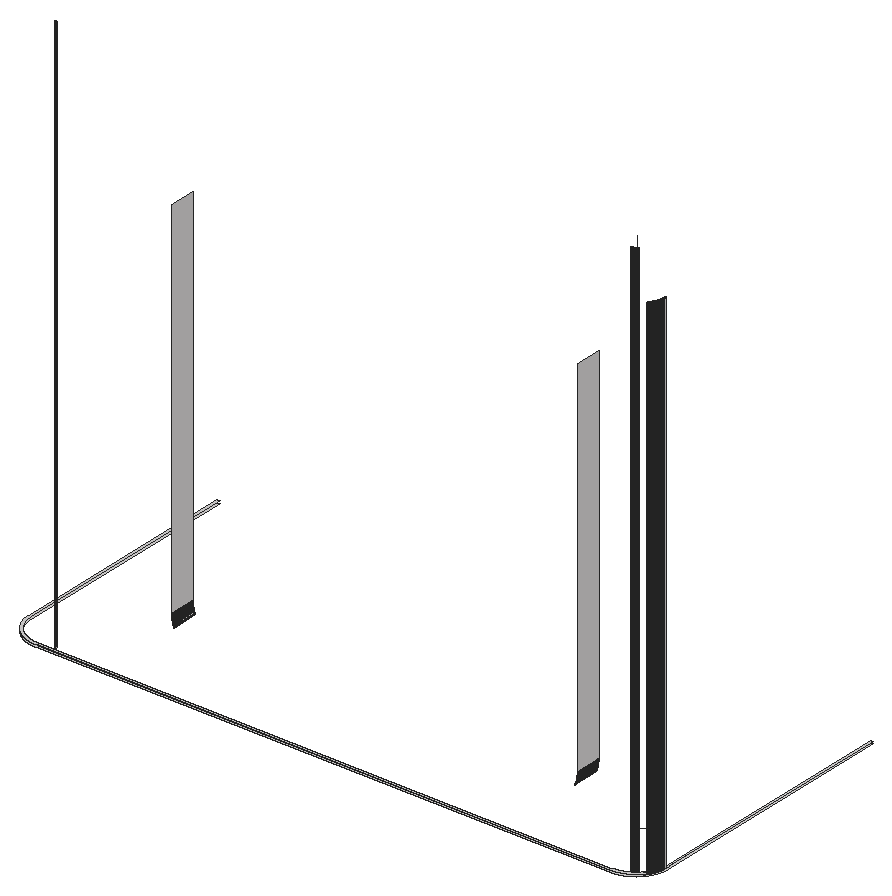
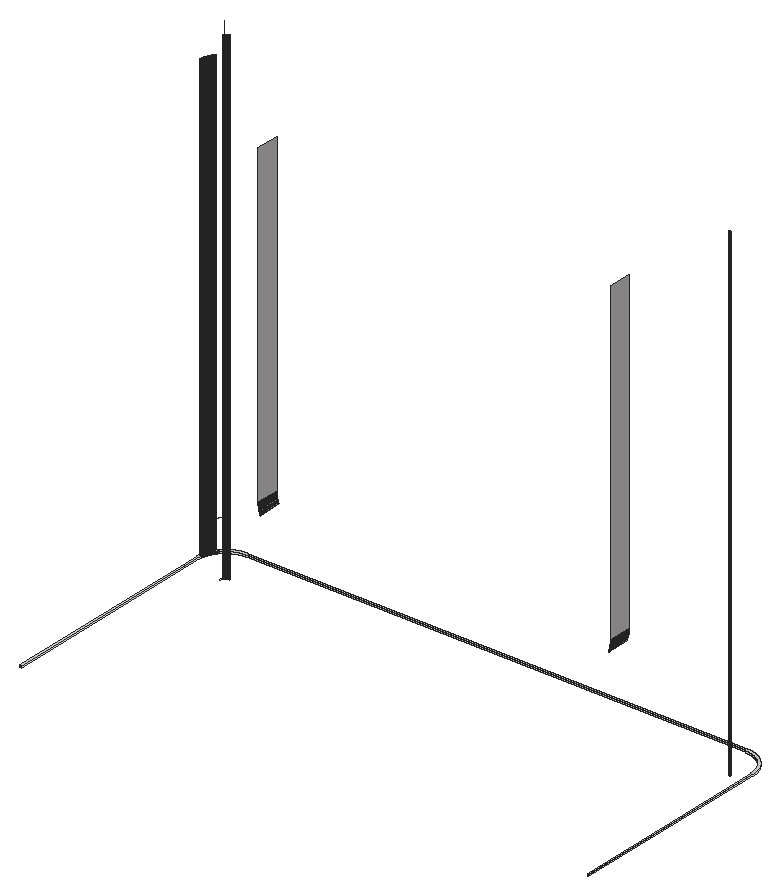
# SketchUp Ruby script. Lengths in inches.
U = 1.inch
M = Sketchup.active_model
def pt(a) = Geom::Point3d.new(a.map { |v| v * U })
def face(e, loops, mat)
  f = e.add_face(loops[0].map { |a| pt(a) })
  loops[1..].each { |l| e.add_face(l.map { |a| pt(a) }).erase! }
  f.material = f.back_material = mat if mat
  f
end
# faces: each face lists its corners as indices into pts; further lists are holes
def faces(e, pts, list, mat = nil) = list.each { |f| face(e, (f[0].is_a?(Array) ? f : [f]).map { |l| l.map { |i| pts[i] } }, mat) }
# xy, xz, yz: faces in a plane at the given z, y or x. An outline is a flat list of corners, or four numbers for a rectangle; further outlines are holes
def ring(l) = l.size == 4 ? [[l[0], l[1]], [l[2], l[1]], [l[2], l[3]], [l[0], l[3]]] : l.each_slice(2).to_a
def flat(e, list, mat, &to3) = list.each { |f| face(e, (f[0].is_a?(Array) ? f : [f]).map { |l| ring(l).map { |u, v| to3.(u, v) } }, mat) }
def xy(e, z, list, mat = nil) = flat(e, list, mat) { |x, y| [x, y, z] }
def xz(e, y, list, mat = nil) = flat(e, list, mat) { |x, z| [x, y, z] }
def yz(e, x, list, mat = nil) = flat(e, list, mat) { |y, z| [x, y, z] }
def lines(e, pts, list) = list.each { |a, b| e.add_line(pt(pts[a]), pt(pts[b])) }
# prism: a flat outline (further loops are holes) pulled along v
def prism(e, loops, v, mat = nil)
  f = face(e, loops, mat); d = Geom::Vector3d.new(v.map { |x| x * U })
  f.pushpull(f.normal.samedirection?(d) ? d.length : -d.length)
end
def box(e, o, s, mat = nil) = prism(e, [[o, [o[0] + s[0], o[1], o[2]], [o[0] + s[0], o[1] + s[1], o[2]], [o[0], o[1] + s[1], o[2]]]], [0, 0, s[2]], mat)
def at(x, y, z, deg = 0) = Geom::Transformation.translation(pt([x, y, z])) * Geom::Transformation.rotation(ORIGIN, Z_AXIS, deg.degrees)
def axes(o, x, y, z) = Geom::Transformation.new([*x, 0, *y, 0, *z, 0, *pt(o).to_a, 1])
def part(name) = M.definitions.add(name)
# library, detail: a bought-in or finely detailed component or shape, given as its bounding box
def library(name, o, s) = part(name).tap { |d| box(d.entities, o, s) }
def detail(e, o, s) = box(e.add_group.entities, o, s)
def put(e, d, t, mat = nil) = e.add_instance(d, t).tap { |i| i.material = mat if mat }
def group(e, t, mat = nil) = e.add_group.tap { |g| g.transformation = t; g.material = mat if mat }.entities
root = M.entities
M.materials.add("[Quartz Light Brown]").color = [215, 212, 212]
xy(root,126,[[480.082,155,480.118,155.002,480.196,155.006,480.235,155.009,480.275,155.013,480.311,155.016,480.314,155.016,480.392,155.026,480.425,155.03,480.43,155.031,480.508,155.043,480.538,155.048,480.547,155.05,480.585,155.058,480.624,155.066,480.651,155.071,480.662,155.074,480.738,155.092,480.762,155.098,480.776,155.102,480.852,155.124,480.873,155.129,480.89,155.135,480.964,155.159,480.982,155.165,481.001,155.172,481.038,155.185,481.075,155.199,481.089,155.204,481.112,155.214,481.148,155.228,481.184,155.244,481.196,155.248,481.22,155.259,481.256,155.276,481.292,155.292,481.3,155.296,481.327,155.309,481.397,155.345,481.402,155.348,481.431,155.364,481.466,155.383,481.5,155.402,481.503,155.403,481.534,155.422,481.567,155.442,481.601,155.463,481.634,155.484,481.697,155.526,481.699,155.528,481.731,155.55,481.763,155.573,481.79,155.592,481.795,155.596,481.857,155.644,481.881,155.663,481.888,155.669,481.918,155.693,481.948,155.719,481.969,155.736,481.978,155.744,482.007,155.771,482.036,155.797,482.054,155.813,482.065,155.824,482.093,155.851,482.121,155.879,482.136,155.893,482.149,155.907,482.176,155.935,482.203,155.964,482.215,155.977,482.229,155.993,482.256,156.022,482.281,156.052,482.291,156.063,482.307,156.082,482.331,156.112,482.356,156.143,482.364,156.152,482.38,156.174,482.404,156.205,482.427,156.237,482.432,156.244,482.45,156.269,482.494,156.333,482.498,156.338,482.516,156.366,482.537,156.399,482.558,156.433,482.56,156.435,482.578,156.466,482.598,156.5,482.617,156.534,482.636,156.569,482.655,156.603,482.672,156.635,482.673,156.638,482.691,156.673,482.708,156.708,482.722,156.738,482.724,156.744,482.741,156.78,482.756,156.816,482.772,156.852,482.786,156.888,482.801,156.925,482.81,156.95,482.815,156.962,482.841,157.036,482.849,157.058,482.853,157.073,482.865,157.11,482.876,157.148,482.882,157.168,482.887,157.186,482.898,157.224,482.908,157.262,482.912,157.279,482.917,157.3,482.926,157.338,482.934,157.376,482.9375,157.391,482.942,157.415,482.95,157.453,482.957,157.492,482.959,157.504,482.963,157.531,482.969,157.57,482.974,157.608,482.976,157.617,482.979,157.647,482.984,157.686,482.987,157.725,482.988,157.731,482.991,157.765,482.994,157.804,482.996,157.843,482.996,157.846,482.998,157.882,482.999,157.921,483,155]],"[Quartz Light Brown]")
xy(root,132,[[216,143,480,143,480.196,143.001,480.393,143.005,480.589,143.012,480.785,143.021,480.981,143.032,481.177,143.046,481.373,143.063,481.568,143.082,481.763,143.104,481.958,143.128,482.152,143.155,482.347,143.185,482.54,143.217,482.734,143.251,482.926,143.288,483.119,143.328,483.31,143.37,483.502,143.414,483.692,143.462,483.882,143.511,484.072,143.563,484.26,143.618,484.448,143.675,484.635,143.734,484.822,143.796,485.007,143.86,485.192,143.927,485.376,143.996,485.558,144.068,485.74,144.142,485.921,144.218,486.101,144.297,486.28,144.378,486.458,144.461,486.634,144.547,486.81,144.635,486.984,144.725,487.157,144.818,487.329,144.913,487.5,145.01,487.669,145.109,487.837,145.21,488.004,145.314,488.17,145.42,488.334,145.528,488.496,145.638,488.657,145.75,488.817,145.865,488.975,145.981,489.131,146.1,489.286,146.22,489.44,146.343,489.592,146.467,489.742,146.594,489.89,146.722,490.037,146.853,490.182,146.985,490.325,147.119,490.467,147.255,490.607,147.393,490.745,147.533,490.881,147.675,491.015,147.818,491.147,147.963,491.278,148.11,491.406,148.258,491.533,148.408,491.657,148.56,491.78,148.714,491.9,148.869,492.019,149.025,492.135,149.183,492.25,149.343,492.362,149.504,492.472,149.666,492.58,149.83,492.686,149.996,492.79,150.163,492.891,150.331,492.99,150.5,493.087,150.671,493.182,150.843,493.275,151.016,493.365,151.19,493.453,151.366,493.539,151.542,493.622,151.72,493.703,151.899,493.782,152.079,493.858,152.26,493.932,152.442,494.004,152.624,494.073,152.808,494.14,152.993,494.204,153.178,494.266,153.365,494.325,153.552,494.382,153.74,494.437,153.928,494.489,154.118,494.538,154.308,494.586,154.498,494.63,154.69,494.672,154.881,494.712,155.074,494.749,155.266,494.783,155.46,494.815,155.653,494.845,155.848,494.872,156.042,494.896,156.237,494.918,156.432,494.937,156.627,494.954,156.823,494.968,157.019,494.979,157.215,494.988,157.411,494.995,157.607,494.999,157.804,495,158,495,275,494,275,494,158.003,493.999,157.817,493.995,157.634,493.989,157.45,493.981,157.267,493.97,157.084,493.957,156.902,493.941,156.719,493.923,156.537,493.903,156.354,493.88,156.173,493.855,155.991,493.828,155.81,493.798,155.629,493.766,155.449,493.731,155.269,493.694,155.089,493.655,154.91,493.613,154.732,493.569,154.554,493.523,154.377,493.474,154.2,493.423,154.024,493.37,153.848,493.315,153.674,493.257,153.5,493.197,153.327,493.135,153.154,493.07,152.983,493.003,152.812,492.934,152.642,492.863,152.474,492.79,152.306,492.714,152.139,492.636,151.973,492.556,151.808,492.474,151.644,492.39,151.481,492.303,151.32,492.215,151.159,492.124,151,492.032,150.842,491.937,150.685,491.84,150.529,491.741,150.375,491.641,150.222,491.538,150.07,491.433,149.92,491.326,149.771,491.218,149.623,491.107,149.477,490.994,149.333,490.88,149.19,490.764,149.048,490.646,148.908,490.526,148.769,490.404,148.632,490.28,148.497,490.155,148.363,490.028,148.231,489.899,148.101,489.769,147.972,489.637,147.845,489.503,147.72,489.368,147.596,489.231,147.474,489.092,147.354,488.952,147.236,488.81,147.12,488.667,147.006,488.523,146.893,488.377,146.782,488.229,146.674,488.08,146.567,487.93,146.462,487.778,146.359,487.625,146.259,487.471,146.16,487.315,146.063,487.158,145.968,487,145.876,486.841,145.785,486.68,145.697,486.519,145.61,486.356,145.526,486.192,145.444,486.027,145.364,485.861,145.286,485.694,145.21,485.526,145.137,485.358,145.066,485.188,144.997,485.017,144.93,484.846,144.865,484.673,144.803,484.5,144.743,484.326,144.685,484.152,144.63,483.976,144.577,483.8,144.526,483.623,144.477,483.446,144.431,483.268,144.387,483.09,144.345,482.911,144.306,482.731,144.269,482.551,144.234,482.371,144.202,482.19,144.172,482.009,144.145,481.827,144.12,481.646,144.097,481.463,144.077,481.281,144.059,481.098,144.043,480.916,144.03,480.733,144.019,480.55,144.011,480.366,144.005,480.183,144.001,479.997,144,216.003,144,215.817,144.001,215.634,144.005,215.45,144.011,215.267,144.019,215.084,144.03,214.902,144.043,214.719,144.059,214.537,144.077,214.354,144.097,214.173,144.12,213.991,144.145,213.81,144.172,213.629,144.202,213.449,144.234,213.269,144.269,213.089,144.306,212.91,144.345,212.732,144.387,212.554,144.431,212.377,144.477,212.2,144.526,212.024,144.577,211.848,144.63,211.674,144.685,211.5,144.743,211.327,144.803,211.154,144.865,210.983,144.93,210.812,144.997,210.642,145.066,210.474,145.137,210.306,145.21,210.139,145.286,209.973,145.364,209.808,145.444,209.644,145.526,209.481,145.61,209.32,145.697,209.159,145.785,209,145.876,208.842,145.968,208.685,146.063,208.529,146.16,208.375,146.259,208.222,146.359,208.07,146.462,207.92,146.567,207.771,146.674,207.623,146.782,207.477,146.893,207.333,147.006,207.19,147.12,207.048,147.236,206.908,147.354,206.769,147.474,206.632,147.596,206.497,147.72,206.363,147.845,206.231,147.972,206.101,148.101,205.972,148.231,205.845,148.363,205.72,148.497,205.596,148.632,205.474,148.769,205.354,148.908,205.236,149.048,205.12,149.19,205.006,149.333,204.893,149.477,204.782,149.623,204.674,149.771,204.567,149.92,204.462,150.07,204.359,150.222,204.259,150.375,204.16,150.529,204.063,150.685,203.968,150.842,203.876,151,203.785,151.159,203.697,151.32,203.61,151.481,203.526,151.644,203.444,151.808,203.364,151.973,203.286,152.139,203.21,152.306,203.137,152.474,203.066,152.642,202.997,152.812,202.93,152.983,202.865,153.154,202.803,153.327,202.743,153.5,202.685,153.674,202.63,153.848,202.577,154.024,202.526,154.2,202.477,154.377,202.431,154.554,202.387,154.732,202.345,154.91,202.306,155.089,202.269,155.269,202.234,155.449,202.202,155.629,202.172,155.81,202.145,155.991,202.12,156.173,202.097,156.354,202.077,156.537,202.059,156.719,202.043,156.902,202.03,157.084,202.019,157.267,202.011,157.45,202.005,157.634,202.001,157.817,202,158.003,202,266,201,266,201,158,201.001,157.804,201.005,157.607,201.012,157.411,201.021,157.215,201.032,157.019,201.046,156.823,201.063,156.627,201.082,156.432,201.104,156.237,201.128,156.042,201.155,155.848,201.185,155.653,201.217,155.46,201.251,155.266,201.288,155.074,201.328,154.881,201.37,154.69,201.414,154.498,201.462,154.308,201.511,154.118,201.563,153.928,201.618,153.74,201.675,153.552,201.734,153.365,201.796,153.178,201.86,152.993,201.927,152.808,201.996,152.624,202.068,152.442,202.142,152.26,202.218,152.079,202.297,151.899,202.378,151.72,202.461,151.542,202.547,151.366,202.635,151.19,202.725,151.016,202.818,150.843,202.913,150.671,203.01,150.5,203.109,150.331,203.21,150.163,203.314,149.996,203.42,149.83,203.528,149.666,203.638,149.504,203.75,149.343,203.865,149.183,203.981,149.025,204.1,148.869,204.22,148.714,204.343,148.56,204.467,148.408,204.594,148.258,204.722,148.11,204.853,147.963,204.985,147.818,205.119,147.675,205.255,147.533,205.393,147.393,205.533,147.255,205.675,147.119,205.818,146.985,205.963,146.853,206.11,146.722,206.258,146.594,206.408,146.467,206.56,146.343,206.714,146.22,206.869,146.1,207.025,145.981,207.183,145.865,207.343,145.75,207.504,145.638,207.666,145.528,207.83,145.42,207.996,145.314,208.163,145.21,208.331,145.109,208.5,145.01,208.671,144.913,208.843,144.818,209.016,144.725,209.19,144.635,209.366,144.547,209.542,144.461,209.72,144.378,209.899,144.297,210.079,144.218,210.26,144.142,210.442,144.068,210.624,143.996,210.808,143.927,210.993,143.86,211.178,143.796,211.365,143.734,211.552,143.675,211.74,143.618,211.928,143.563,212.118,143.511,212.308,143.462,212.498,143.414,212.69,143.37,212.881,143.328,213.074,143.288,213.266,143.251,213.46,143.217,213.653,143.185,213.848,143.155,214.042,143.128,214.237,143.104,214.432,143.082,214.627,143.063,214.823,143.046,215.019,143.032,215.215,143.021,215.411,143.012,215.607,143.005,215.804,143.001]],"[Quartz Light Brown]")
xy(root,133,[[216,143,215.804,143.001,215.607,143.005,215.411,143.012,215.215,143.021,215.019,143.032,214.823,143.046,214.627,143.063,214.432,143.082,214.237,143.104,214.042,143.128,213.848,143.155,213.653,143.185,213.46,143.217,213.266,143.251,213.074,143.288,212.881,143.328,212.69,143.37,212.498,143.414,212.308,143.462,212.118,143.511,211.928,143.563,211.74,143.618,211.552,143.675,211.365,143.734,211.178,143.796,210.993,143.86,210.808,143.927,210.624,143.996,210.442,144.068,210.26,144.142,210.079,144.218,209.899,144.297,209.72,144.378,209.542,144.461,209.366,144.547,209.19,144.635,209.016,144.725,208.843,144.818,208.671,144.913,208.5,145.01,208.331,145.109,208.163,145.21,207.996,145.314,207.83,145.42,207.666,145.528,207.504,145.638,207.343,145.75,207.183,145.865,207.025,145.981,206.869,146.1,206.714,146.22,206.56,146.343,206.408,146.467,206.258,146.594,206.11,146.722,205.963,146.853,205.818,146.985,205.675,147.119,205.533,147.255,205.393,147.393,205.255,147.533,205.119,147.675,204.985,147.818,204.853,147.963,204.722,148.11,204.594,148.258,204.467,148.408,204.343,148.56,204.22,148.714,204.1,148.869,203.981,149.025,203.865,149.183,203.75,149.343,203.638,149.504,203.528,149.666,203.42,149.83,203.314,149.996,203.21,150.163,203.109,150.331,203.01,150.5,202.913,150.671,202.818,150.843,202.725,151.016,202.635,151.19,202.547,151.366,202.461,151.542,202.378,151.72,202.297,151.899,202.218,152.079,202.142,152.26,202.068,152.442,201.996,152.624,201.927,152.808,201.86,152.993,201.796,153.178,201.734,153.365,201.675,153.552,201.618,153.74,201.563,153.928,201.511,154.118,201.462,154.308,201.414,154.498,201.37,154.69,201.328,154.881,201.288,155.074,201.251,155.266,201.217,155.46,201.185,155.653,201.155,155.848,201.128,156.042,201.104,156.237,201.082,156.432,201.063,156.627,201.046,156.823,201.032,157.019,201.021,157.215,201.012,157.411,201.005,157.607,201.001,157.804,201,158,201,266,202,266,202,158.003,202.001,157.817,202.005,157.634,202.011,157.45,202.019,157.267,202.03,157.084,202.043,156.902,202.059,156.719,202.077,156.537,202.097,156.354,202.12,156.173,202.145,155.991,202.172,155.81,202.202,155.629,202.234,155.449,202.269,155.269,202.306,155.089,202.345,154.91,202.387,154.732,202.431,154.554,202.477,154.377,202.526,154.2,202.577,154.024,202.63,153.848,202.685,153.674,202.743,153.5,202.803,153.327,202.865,153.154,202.93,152.983,202.997,152.812,203.066,152.642,203.137,152.474,203.21,152.306,203.286,152.139,203.364,151.973,203.444,151.808,203.526,151.644,203.61,151.481,203.697,151.32,203.785,151.159,203.876,151,203.968,150.842,204.063,150.685,204.16,150.529,204.259,150.375,204.359,150.222,204.462,150.07,204.567,149.92,204.674,149.771,204.782,149.623,204.893,149.477,205.006,149.333,205.12,149.19,205.236,149.048,205.354,148.908,205.474,148.769,205.596,148.632,205.72,148.497,205.845,148.363,205.972,148.231,206.101,148.101,206.231,147.972,206.363,147.845,206.497,147.72,206.632,147.596,206.769,147.474,206.908,147.354,207.048,147.236,207.19,147.12,207.333,147.006,207.477,146.893,207.623,146.782,207.771,146.674,207.92,146.567,208.07,146.462,208.222,146.359,208.375,146.259,208.529,146.16,208.685,146.063,208.842,145.968,209,145.876,209.159,145.785,209.32,145.697,209.481,145.61,209.644,145.526,209.808,145.444,209.973,145.364,210.139,145.286,210.306,145.21,210.474,145.137,210.642,145.066,210.812,144.997,210.983,144.93,211.154,144.865,211.327,144.803,211.5,144.743,211.674,144.685,211.848,144.63,212.024,144.577,212.2,144.526,212.377,144.477,212.554,144.431,212.732,144.387,212.91,144.345,213.089,144.306,213.269,144.269,213.449,144.234,213.629,144.202,213.81,144.172,213.991,144.145,214.173,144.12,214.354,144.097,214.537,144.077,214.719,144.059,214.902,144.043,215.084,144.03,215.267,144.019,215.45,144.011,215.634,144.005,215.817,144.001,216.003,144,479.997,144,480.183,144.001,480.366,144.005,480.55,144.011,480.733,144.019,480.916,144.03,481.098,144.043,481.281,144.059,481.463,144.077,481.646,144.097,481.827,144.12,482.009,144.145,482.19,144.172,482.371,144.202,482.551,144.234,482.731,144.269,482.911,144.306,483.09,144.345,483.268,144.387,483.446,144.431,483.623,144.477,483.8,144.526,483.976,144.577,484.152,144.63,484.326,144.685,484.5,144.743,484.673,144.803,484.846,144.865,485.017,144.93,485.188,144.997,485.358,145.066,485.526,145.137,485.694,145.21,485.861,145.286,486.027,145.364,486.192,145.444,486.356,145.526,486.519,145.61,486.68,145.697,486.841,145.785,487,145.876,487.158,145.968,487.315,146.063,487.471,146.16,487.625,146.259,487.778,146.359,487.93,146.462,488.08,146.567,488.229,146.674,488.377,146.782,488.523,146.893,488.667,147.006,488.81,147.12,488.952,147.236,489.092,147.354,489.231,147.474,489.368,147.596,489.503,147.72,489.637,147.845,489.769,147.972,489.899,148.101,490.028,148.231,490.155,148.363,490.28,148.497,490.404,148.632,490.526,148.769,490.646,148.908,490.764,149.048,490.88,149.19,490.994,149.333,491.107,149.477,491.218,149.623,491.326,149.771,491.433,149.92,491.538,150.07,491.641,150.222,491.741,150.375,491.84,150.529,491.937,150.685,492.032,150.842,492.124,151,492.215,151.159,492.303,151.32,492.39,151.481,492.474,151.644,492.556,151.808,492.636,151.973,492.714,152.139,492.79,152.306,492.863,152.474,492.934,152.642,493.003,152.812,493.07,152.983,493.135,153.154,493.197,153.327,493.257,153.5,493.315,153.674,493.37,153.848,493.423,154.024,493.474,154.2,493.523,154.377,493.569,154.554,493.613,154.732,493.655,154.91,493.694,155.089,493.731,155.269,493.766,155.449,493.798,155.629,493.828,155.81,493.855,155.991,493.88,156.173,493.903,156.354,493.923,156.537,493.941,156.719,493.957,156.902,493.97,157.084,493.981,157.267,493.989,157.45,493.995,157.634,493.999,157.817,494,158.003,494,275,495,275,495,158,494.999,157.804,494.995,157.607,494.988,157.411,494.979,157.215,494.968,157.019,494.954,156.823,494.937,156.627,494.918,156.432,494.896,156.237,494.872,156.042,494.845,155.848,494.815,155.653,494.783,155.46,494.749,155.266,494.712,155.074,494.672,154.881,494.63,154.69,494.586,154.498,494.538,154.308,494.489,154.118,494.437,153.928,494.382,153.74,494.325,153.552,494.266,153.365,494.204,153.178,494.14,152.993,494.073,152.808,494.004,152.624,493.932,152.442,493.858,152.26,493.782,152.079,493.703,151.899,493.622,151.72,493.539,151.542,493.453,151.366,493.365,151.19,493.275,151.016,493.182,150.843,493.087,150.671,492.99,150.5,492.891,150.331,492.79,150.163,492.686,149.996,492.58,149.83,492.472,149.666,492.362,149.504,492.25,149.343,492.135,149.183,492.019,149.025,491.9,148.869,491.78,148.714,491.657,148.56,491.533,148.408,491.406,148.258,491.278,148.11,491.147,147.963,491.015,147.818,490.881,147.675,490.745,147.533,490.607,147.393,490.467,147.255,490.325,147.119,490.182,146.985,490.037,146.853,489.89,146.722,489.742,146.594,489.592,146.467,489.44,146.343,489.286,146.22,489.131,146.1,488.975,145.981,488.817,145.865,488.657,145.75,488.496,145.638,488.334,145.528,488.17,145.42,488.004,145.314,487.837,145.21,487.669,145.109,487.5,145.01,487.329,144.913,487.157,144.818,486.984,144.725,486.81,144.635,486.634,144.547,486.458,144.461,486.28,144.378,486.101,144.297,485.921,144.218,485.74,144.142,485.558,144.068,485.376,143.996,485.192,143.927,485.007,143.86,484.822,143.796,484.635,143.734,484.448,143.675,484.26,143.618,484.072,143.563,483.882,143.511,483.692,143.462,483.502,143.414,483.31,143.37,483.119,143.328,482.926,143.288,482.734,143.251,482.54,143.217,482.347,143.185,482.152,143.155,481.958,143.128,481.763,143.104,481.568,143.082,481.373,143.063,481.177,143.046,480.981,143.032,480.785,143.021,480.589,143.012,480.393,143.005,480.196,143.001,480,143]],"[Quartz Light Brown]")
xz(root,155.002,[[215.879,126,215.882,384]],"[Quartz Light Brown]")
xz(root,155.021,[[215.644,126,215.647,384]],"[Quartz Light Brown]")
xz(root,155.037,[[215.528,126,215.531,384]],"[Quartz Light Brown]")
xz(root,155.058,[[215.412,126,215.415,384]],"[Quartz Light Brown]")
xz(root,155.113,[[215.183,126,215.186,384]],"[Quartz Light Brown]")
yz(root,278.5,[[143,168,155,336]],"[Quartz Light Brown]")
yz(root,465,[[143,168,155,336]],"[Quartz Light Brown]")
p = [[215.453,155.05,384],[215.492,155.043,384],[215.492,155.043,126],[215.453,155.05,126],[215.528,155.037,384],[215.528,155.037,126],
  [215.531,155.037,384],[215.57,155.031,384],[215.57,155.031,126],[215.531,155.037,126],[215.608,155.026,384],[215.608,155.026,126],
  [215.644,155.021,384],[215.644,155.021,126],[215.647,155.021,384],[215.686,155.016,384],[215.686,155.016,126],[215.647,155.021,126],
  [215.725,155.013,384],[215.725,155.013,126],[215.761,155.01,384],[215.761,155.01,126],[215.765,155.009,126],[215.765,155.009,384],
  [215.804,155.006,384],[215.804,155.006,126],[215.843,155.004,384],[215.843,155.004,126],[215.879,155.002,384],[215.879,155.002,126],
  [215.882,155.002,384],[215.921,155.001,384],[215.921,155.001,126],[215.882,155.002,126],[480.079,155.001,384],[480.082,155,384],
  [480.082,155,126],[480.079,155,126],[480.118,155.002,126],[480.118,155.002,384],[480.157,155.004,384],[480.157,155.004,126],
  [480.196,155.006,384],[480.196,155.006,126],[480.235,155.009,384],[480.235,155.009,126],[480.275,155.013,384],[480.275,155.013,126],
  [480.311,155.015,384],[480.311,155.016,126],[480.314,155.016,126],[480.314,155.016,384],[480.353,155.021,384],[480.353,155.021,126],
  [480.392,155.026,384],[480.392,155.026,126],[480.425,155.029,384],[480.425,155.03,126],[480.43,155.031,126],[480.43,155.031,384],
  [480.469,155.037,384],[480.469,155.037,126],[480.508,155.043,384],[480.508,155.043,126],[480.538,155.048,384],[480.538,155.048,126],
  [480.547,155.05,126],[480.547,155.05,384],[215.036,155.159,384],[215.07,155.148,384],[215.07,155.148,126],[215.036,155.159,126],
  [215.073,155.147,126],[215.073,155.147,384],[215.11,155.135,384],[215.11,155.135,126],[215.148,155.124,384],[215.148,155.124,126],
  [215.183,155.113,384],[215.183,155.113,126],[215.186,155.113,384],[215.224,155.102,384],[215.224,155.102,126],[215.186,155.113,126],
  [215.262,155.092,384],[215.262,155.092,126],[215.297,155.084,384],[215.297,155.084,126],[215.3,155.083,126],[215.3,155.083,384],
  [215.338,155.074,384],[215.338,155.074,126],[215.376,155.066,384],[215.376,155.066,126],[215.412,155.058,384],[215.412,155.058,126],
  [215.415,155.058,384],[215.415,155.058,126],[480.585,155.058,384],[480.585,155.058,126],[480.624,155.066,384],[480.624,155.066,126],
  [480.651,155.071,384],[480.651,155.071,126],[480.662,155.074,126],[480.662,155.074,384],[480.7,155.083,384],[480.7,155.083,126],
  [480.738,155.092,384],[480.738,155.092,126],[480.762,155.098,384],[480.762,155.098,126],[480.776,155.102,126],[480.776,155.102,384],
  [480.814,155.113,384],[480.814,155.113,126],[480.852,155.124,384],[480.852,155.124,126],[480.873,155.129,384],[480.873,155.129,126],
  [480.89,155.135,126],[480.89,155.135,384],[480.927,155.147,384],[480.927,155.147,126],[480.964,155.159,384],[480.964,155.159,126],
  [214.816,155.244,384],[214.85,155.229,384],[214.85,155.229,126],[214.816,155.244,126],[214.852,155.228,126],[214.852,155.228,384],
  [214.888,155.214,384],[214.888,155.214,126],[214.925,155.199,384],[214.925,155.199,126],[214.959,155.186,384],[214.959,155.186,126],
  [214.962,155.185,126],[214.962,155.185,384],[214.999,155.172,384],[214.999,155.172,126],[480.982,155.164,384],[480.982,155.165,126],
  [481.001,155.172,126],[481.001,155.172,384],[481.038,155.185,384],[481.038,155.185,126],[481.075,155.199,384],[481.075,155.199,126],
  [481.09,155.204,384],[481.089,155.204,126],[481.112,155.214,126],[481.112,155.214,384],[481.148,155.228,384],[481.148,155.228,126],
  [481.184,155.244,384],[481.184,155.244,126],[481.196,155.248,384],[481.196,155.248,126],[481.22,155.259,126],[481.22,155.259,384],
  [481.256,155.276,384],[481.256,155.276,126],[481.292,155.292,384],[481.292,155.292,126],[481.3,155.295,384],[481.3,155.296,126],
  [481.327,155.309,126],[481.327,155.309,384],[481.362,155.327,384],[481.362,155.327,126],[481.397,155.345,384],[481.397,155.345,126],
  [481.403,155.347,384],[481.402,155.348,126],[481.431,155.364,126],[481.431,155.364,384],[481.466,155.383,384],[481.466,155.383,126],
  [481.5,155.402,384],[481.5,155.402,126],[481.503,155.403,384],[481.503,155.403,126],[481.534,155.422,126],[481.534,155.422,384],
  [481.567,155.442,384],[481.567,155.442,126],[481.601,155.463,384],[481.601,155.463,126],[481.634,155.484,384],[481.634,155.484,126],
  [481.667,155.506,384],[481.667,155.506,126],[481.697,155.525,384],[481.697,155.526,126],[481.699,155.528,126],[481.699,155.528,384],
  [481.731,155.55,384],[481.731,155.55,126],[481.763,155.573,384],[481.763,155.573,126],[481.791,155.592,384],[481.79,155.592,126],
  [481.795,155.596,126],[481.795,155.596,384],[481.826,155.62,384],[481.826,155.62,126],[481.857,155.644,384],[481.857,155.644,126],
  [481.881,155.662,384],[481.881,155.663,126],[481.888,155.669,126],[481.888,155.669,384],[481.918,155.693,384],[481.918,155.693,126],
  [481.948,155.719,384],[481.948,155.719,126],[481.969,155.736,384],[481.969,155.736,126],[481.978,155.744,126],[481.978,155.744,384],
  [482.007,155.771,384],[482.007,155.771,126],[482.036,155.797,384],[482.036,155.797,126],[482.054,155.813,384],[482.054,155.813,126],
  [482.065,155.824,126],[482.065,155.824,384],[482.093,155.851,384],[482.093,155.851,126],[482.121,155.879,384],[482.121,155.879,126],
  [482.137,155.893,384],[482.136,155.893,126],[482.149,155.907,126],[482.149,155.907,384],[482.176,155.935,384],[482.176,155.935,126],
  [482.203,155.964,384],[482.203,155.964,126],[482.216,155.976,384],[482.215,155.977,126],[482.229,155.993,126],[482.229,155.993,384],
  [482.256,156.022,384],[482.256,156.022,126],[482.281,156.052,384],[482.281,156.052,126],[482.291,156.063,384],[482.291,156.063,126],
  [482.307,156.082,126],[482.307,156.082,384],[482.329,156.109,384],[482.331,156.112,384],[482.331,156.112,126],[482.333,156.114,384],
  [482.356,156.143,384],[482.356,156.143,126],[482.364,156.152,384],[482.364,156.152,126],[482.38,156.174,126],[482.38,156.174,384],
  [482.397,156.196,384],[482.404,156.205,384],[482.404,156.205,126],[482.406,156.209,384],[482.427,156.237,384],[482.427,156.237,126],
  [482.433,156.244,384],[482.432,156.244,126],[482.45,156.269,126],[482.45,156.269,384],[482.46,156.283,384],[482.472,156.301,384],
  [482.472,156.301,126],[482.476,156.306,384],[482.494,156.333,384],[482.494,156.333,126],[490.764,149.048,133],[490.764,149.048,132],
  [490.88,149.19,132],[490.88,149.19,133],[490.994,149.333,132],[490.994,149.333,133],[491.107,149.477,132],[491.107,149.477,133],
  [491.218,149.623,132],[491.218,149.623,133],[491.326,149.771,132],[491.326,149.771,133],[491.433,149.92,132],[491.433,149.92,133],
  [491.538,150.07,132],[491.538,150.07,133],[491.641,150.222,132],[491.641,150.222,133],[491.741,150.375,132],[491.741,150.375,133],
  [491.84,150.529,132],[491.84,150.529,133],[491.937,150.685,132],[491.937,150.685,133],[492.032,150.842,132],[492.032,150.842,133],
  [492.124,151,132],[492.124,151,133],[492.215,151.159,132],[492.215,151.159,133],[492.303,151.32,132],[492.303,151.32,133],
  [492.39,151.481,132],[492.39,151.481,133],[492.474,151.644,132],[492.474,151.644,133],[492.556,151.808,132],[492.556,151.808,133],
  [492.636,151.973,132],[492.636,151.973,133],[492.714,152.139,132],[492.714,152.139,133],[492.79,152.306,132],[492.79,152.306,133],
  [492.863,152.474,132],[492.863,152.474,133],[492.934,152.642,132],[492.934,152.642,133],[493.003,152.812,132],[493.003,152.812,133],
  [493.07,152.983,132],[493.07,152.983,133],[493.135,153.154,132],[493.135,153.154,133],[493.197,153.327,132],[493.197,153.327,133],
  [493.257,153.5,132],[493.257,153.5,133],[493.315,153.674,132],[493.315,153.674,133],[493.37,153.848,132],[493.37,153.848,133],
  [493.423,154.024,132],[493.423,154.024,133],[493.474,154.2,132],[493.474,154.2,133],[493.523,154.377,132],[493.523,154.377,133],
  [493.569,154.554,132],[493.569,154.554,133],[493.613,154.732,132],[493.613,154.732,133],[493.655,154.91,132],[493.655,154.91,133],
  [493.694,155.089,132],[493.694,155.089,133],[493.731,155.269,132],[493.731,155.269,133],[493.766,155.449,132],[493.766,155.449,133],
  [493.798,155.629,132],[493.798,155.629,133],[493.828,155.81,132],[493.828,155.81,133],[493.855,155.991,132],[493.855,155.991,133],
  [493.88,156.173,132],[493.88,156.173,133],[493.903,156.354,132],[493.903,156.354,133],[492.019,149.025,368],[492.019,149.025,133],
  [492.135,149.183,133],[492.135,149.183,368],[492.25,149.343,133],[492.25,149.343,368],[492.362,149.504,133],[492.362,149.504,368],
  [492.472,149.666,133],[492.472,149.666,368],[492.58,149.83,133],[492.58,149.83,368],[492.686,149.996,133],[492.686,149.996,368],
  [492.79,150.163,133],[492.79,150.163,368],[492.891,150.331,133],[492.891,150.331,368],[492.99,150.5,133],[492.99,150.5,368],
  [493.087,150.671,133],[493.087,150.671,368],[493.182,150.843,133],[493.182,150.843,368],[493.275,151.016,133],[493.275,151.016,368],
  [493.365,151.19,133],[493.365,151.19,368],[493.453,151.366,133],[493.453,151.366,368],[493.539,151.542,133],[493.539,151.542,368],
  [493.622,151.72,133],[493.622,151.72,368],[493.703,151.899,133],[493.703,151.899,368],[493.782,152.079,133],[493.782,152.079,368],
  [493.858,152.26,133],[493.858,152.26,368],[493.932,152.442,133],[493.932,152.442,368],[494.004,152.624,133],[494.004,152.624,368],
  [494.073,152.808,133],[494.073,152.808,368],[494.14,152.993,133],[494.14,152.993,368],[494.204,153.178,133],[494.204,153.178,368],
  [494.266,153.365,133],[494.266,153.365,368],[494.325,153.552,133],[494.325,153.552,368],[494.382,153.74,133],[494.382,153.74,368],
  [494.437,153.928,133],[494.437,153.928,368],[494.489,154.118,133],[494.489,154.118,368],[494.538,154.308,133],[494.538,154.308,368],
  [494.586,154.498,133],[494.586,154.498,368],[494.63,154.69,133],[494.63,154.69,368],[494.672,154.881,133],[494.672,154.881,368],
  [494.712,155.074,133],[494.712,155.074,368],[494.749,155.266,133],[494.749,155.266,368],[494.783,155.46,133],[494.783,155.46,368],
  [494.815,155.653,133],[494.815,155.653,368],[494.845,155.848,133],[494.845,155.848,368],[494.872,156.042,133],[494.872,156.042,368],
  [494.896,156.237,133],[494.896,156.237,368],[279.642,143,162.26],[279.718,143,162.079],[279.718,155,162.079],[279.642,155,162.26],
  [463.782,143,162.079],[463.858,143,162.26],[463.858,155,162.26],[463.782,155,162.079],[279.568,143,162.442],[279.568,155,162.442],
  [463.932,143,162.442],[463.932,155,162.442],[279.496,143,162.624],[279.496,155,162.624],[464.004,143,162.624],[464.004,155,162.624],
  [279.427,143,162.808],[279.427,155,162.808],[464.073,143,162.808],[464.073,155,162.808],[279.36,143,162.993],[279.36,155,162.993],
  [464.14,143,162.993],[464.14,155,162.993],[279.296,143,163.178],[279.296,155,163.178],[464.204,143,163.178],[464.204,155,163.178],
  [279.234,143,163.365],[279.234,155,163.365],[464.266,143,163.365],[464.266,155,163.365],[279.175,143,163.552],[279.175,155,163.552],
  [464.325,143,163.552],[464.325,155,163.552],[279.118,143,163.74],[279.118,155,163.74],[464.382,143,163.74],[464.382,155,163.74],
  [279.063,143,163.928],[279.063,155,163.928],[464.437,143,163.928],[464.437,155,163.928],[279.011,143,164.118],[279.011,155,164.118],
  [464.489,143,164.118],[464.489,155,164.118],[278.962,143,164.308],[278.962,155,164.308],[464.538,143,164.308],[464.538,155,164.308],
  [278.914,143,164.498],[278.914,155,164.498],[464.586,143,164.498],[464.586,155,164.498],[278.87,143,164.69],[278.87,155,164.69],
  [464.63,143,164.69],[464.63,155,164.69],[278.828,143,164.881],[278.828,155,164.881],[464.672,143,164.881],[464.672,155,164.881],
  [278.788,143,165.074],[278.788,155,165.074],[464.712,143,165.074],[464.712,155,165.074],[278.751,143,165.266],[278.751,155,165.266],
  [464.749,143,165.266],[464.749,155,165.266],[278.717,143,165.46],[278.717,155,165.46],[464.783,143,165.46],[464.783,155,165.46],
  [278.685,143,165.653],[278.685,155,165.653],[464.815,143,165.653],[464.815,155,165.653],[278.655,143,165.848],[278.655,155,165.848],
  [464.845,143,165.848],[464.845,155,165.848],[278.628,143,166.042],[278.628,155,166.042],[464.872,143,166.042],[464.872,155,166.042],
  [278.604,143,166.237],[278.604,155,166.237],[464.896,143,166.237],[464.896,155,166.237],[278.582,143,166.432],[278.582,155,166.432],
  [464.918,143,166.432],[464.918,155,166.432],[278.563,143,166.627],[278.563,155,166.627],[464.937,143,166.627],[464.937,155,166.627],
  [278.546,143,166.823],[278.546,155,166.823],[464.954,143,166.823],[464.954,155,166.823],[278.532,143,167.019],[278.532,155,167.019],
  [464.968,143,167.019],[464.968,155,167.019],[278.521,143,167.215],[278.521,155,167.215],[464.979,143,167.215],[464.979,155,167.215],
  [278.512,143,167.411],[278.512,155,167.411],[464.988,143,167.411],[464.988,155,167.411],[278.505,143,167.607],[278.505,155,167.607],
  [464.995,143,167.607],[464.995,155,167.607],[278.501,143,167.804],[278.501,155,167.804],[464.999,143,167.804],[464.999,155,167.804],
  [278.5,143,168],[278.5,155,168],[465,143,168],[465,155,168],[487.912,148.978,150],[488.03,149.082,150],
  [488.146,149.188,150],[488.26,149.296,150],[488.373,149.404,150],[488.485,149.515,150],[488.596,149.627,150],[488.704,149.74,150],
  [488.812,149.854,150],[488.918,149.97,150],[489.022,150.088,150],[489.125,150.207,150],[489.226,150.327,150],[489.326,150.448,150],
  [489.424,150.571,150],[489.52,150.695,150],[489.615,150.82,150],[489.708,150.947,150],[489.8,151.074,150],[489.89,151.203,150],
  [489.978,151.333,150],[490.064,151.464,150],[490.149,151.597,150],[490.232,151.73,150],[490.313,151.864,150],[490.392,152,150],
  [490.47,152.137,150],[490.546,152.274,150],[490.62,152.413,150],[490.692,152.552,150],[490.762,152.693,150],[490.831,152.834,150],
  [490.898,152.976,150],[490.963,153.119,150],[491.025,153.263,150],[491.087,153.408,150],[491.146,153.553,150],[491.203,153.7,150],
  [491.258,153.847,150],[491.312,153.994,150],[491.363,154.143,150],[491.413,154.292,150],[491.46,154.442,150],[491.506,154.592,150],
  [491.549,154.743,150],[491.591,154.894,150],[491.631,155.046,150],[491.668,155.199,150],[491.704,155.352,150],[491.738,155.505,150],
  [491.769,155.659,150],[491.799,155.813,150],[491.827,155.968,150],[491.852,156.123,150],[491.876,156.278,150],[483,155,126],
  [483,155,390]]
faces(root,p,[[0,1,2,3],[1,4,5,2],[6,7,8,9],[7,10,11,8],[10,12,13,11],[14,15,16,17],[15,18,19,16],[18,20,21,19],
  [22,21,20,23],[23,24,25,22],[24,26,27,25],[26,28,29,27],[30,31,32,33],[34,35,36,37],[38,36,35,39],[39,40,41,38],
  [40,42,43,41],[42,44,45,43],[44,46,47,45],[46,48,49,47],[50,49,48,51],[51,52,53,50],[52,54,55,53],[54,56,57,55],
  [58,57,56,59],[59,60,61,58],[60,62,63,61],[62,64,65,63],[66,65,64,67],[68,69,70,71],[72,70,69,73],[73,74,75,72],
  [74,76,77,75],[76,78,79,77],[80,81,82,83],[81,84,85,82],[84,86,87,85],[88,87,86,89],[89,90,91,88],[90,92,93,91],
  [92,94,95,93],[96,0,3,97],[67,98,99,66],[98,100,101,99],[100,102,103,101],[104,103,102,105],[105,106,107,104],[106,108,109,107],
  [108,110,111,109],[112,111,110,113],[113,114,115,112],[114,116,117,115],[116,118,119,117],[120,119,118,121],[121,122,123,120],[122,124,125,123],
  [126,127,128,129],[130,128,127,131],[131,132,133,130],[132,134,135,133],[134,136,137,135],[138,137,136,139],[139,140,141,138],[140,68,71,141],
  [124,142,143,125],[144,143,142,145],[145,146,147,144],[146,148,149,147],[148,150,151,149],[152,151,150,153],[153,154,155,152],[154,156,157,155],
  [156,158,159,157],[160,159,158,161],[161,162,163,160],[162,164,165,163],[164,166,167,165],[168,167,166,169],[169,170,171,168],[170,172,173,171],
  [172,174,175,173],[176,175,174,177],[177,178,179,176],[178,180,181,179],[180,182,183,181],[184,183,182,185],[185,186,187,184],[186,188,189,187],
  [188,190,191,189],[190,192,193,191],[192,194,195,193],[196,195,194,197],[197,198,199,196],[198,200,201,199],[200,202,203,201],[204,203,202,205],
  [205,206,207,204],[206,208,209,207],[208,210,211,209],[212,211,210,213],[213,214,215,212],[214,216,217,215],[216,218,219,217],[220,219,218,221],
  [221,222,223,220],[222,224,225,223],[224,226,227,225],[228,227,226,229],[229,230,231,228],[230,232,233,231],[232,234,235,233],[236,235,234,237],
  [237,238,239,236],[238,240,241,239],[240,242,243,241],[244,243,242,245],[245,246,247,244],[246,248,249,247],[248,250,251,249],[252,251,250,253],
  [253,254,255,256,252],[255,257,258,259,256],[258,260,261,259],[262,261,260,263],[263,264,265,266,262],[265,267,268,269,266],[268,270,271,269],[272,271,270,273],
  [273,274,275,276,272],[275,277,278,279,276],[280,281,282,283],[283,282,284,285],[285,284,286,287],[287,286,288,289],[289,288,290,291],[291,290,292,293],
  [293,292,294,295],[295,294,296,297],[297,296,298,299],[299,298,300,301],[301,300,302,303],[303,302,304,305],[305,304,306,307],[307,306,308,309],
  [309,308,310,311],[311,310,312,313],[313,312,314,315],[315,314,316,317],[317,316,318,319],[319,318,320,321],[321,320,322,323],[323,322,324,325],
  [325,324,326,327],[327,326,328,329],[329,328,330,331],[331,330,332,333],[333,332,334,335],[335,334,336,337],[337,336,338,339],[339,338,340,341],
  [341,340,342,343],[343,342,344,345],[345,344,346,347],[347,346,348,349],[349,348,350,351],[351,350,352,353],[353,352,354,355],[355,354,356,357],
  [357,356,358,359],[359,358,360,361],[361,360,362,363],[363,362,364,365],[365,364,366,367],[367,366,368,369],[370,371,372,373],[373,372,374,375],
  [375,374,376,377],[377,376,378,379],[379,378,380,381],[381,380,382,383],[383,382,384,385],[385,384,386,387],[387,386,388,389],[389,388,390,391],
  [391,390,392,393],[393,392,394,395],[395,394,396,397],[397,396,398,399],[399,398,400,401],[401,400,402,403],[403,402,404,405],[405,404,406,407],
  [407,406,408,409],[409,408,410,411],[411,410,412,413],[413,412,414,415],[415,414,416,417],[417,416,418,419],[419,418,420,421],[421,420,422,423],
  [423,422,424,425],[425,424,426,427],[427,426,428,429],[429,428,430,431],[431,430,432,433],[433,432,434,435],[435,434,436,437],[437,436,438,439],
  [439,438,440,441],[441,440,442,443],[443,442,444,445],[445,444,446,447],[447,446,448,449],[449,448,450,451],[452,453,454,455],[456,457,458,459],
  [460,452,455,461],[457,462,463,458],[464,460,461,465],[462,466,467,463],[468,464,465,469],[466,470,471,467],[472,468,469,473],[470,474,475,471],
  [476,472,473,477],[474,478,479,475],[480,476,477,481],[478,482,483,479],[484,480,481,485],[482,486,487,483],[488,484,485,489],[486,490,491,487],
  [492,488,489,493],[490,494,495,491],[496,492,493,497],[494,498,499,495],[500,496,497,501],[498,502,503,499],[504,500,501,505],[502,506,507,503],
  [508,504,505,509],[506,510,511,507],[512,508,509,513],[510,514,515,511],[516,512,513,517],[514,518,519,515],[520,516,517,521],[518,522,523,519],
  [524,520,521,525],[522,526,527,523],[528,524,525,529],[526,530,531,527],[532,528,529,533],[530,534,535,531],[536,532,533,537],[534,538,539,535],
  [540,536,537,541],[538,542,543,539],[544,540,541,545],[542,546,547,543],[548,544,545,549],[546,550,551,547],[552,548,549,553],[550,554,555,551],
  [556,552,553,557],[554,558,559,555],[560,556,557,561],[558,562,563,559],[564,560,561,565],[562,566,567,563],[568,564,565,569],[566,570,571,567],
  [572,568,569,573],[570,574,575,571],[576,572,573,577],[574,578,579,575]],"[Quartz Light Brown]")
lines(root,p,[[580,581],[581,582],[582,583],[583,584],[584,585],[585,586],[586,587],[587,588],[588,589],[589,590],[590,591],[591,592],
  [592,593],[593,594],[594,595],[595,596],[596,597],[597,598],[598,599],[599,600],[600,601],[601,602],[602,603],[603,604],
  [604,605],[605,606],[606,607],[607,608],[608,609],[609,610],[610,611],[611,612],[612,613],[613,614],[614,615],[615,616],
  [616,617],[617,618],[618,619],[619,620],[620,621],[621,622],[622,623],[623,624],[624,625],[625,626],[626,627],[627,628],
  [628,629],[629,630],[630,631],[631,632],[632,633],[633,634],[635,636]])
